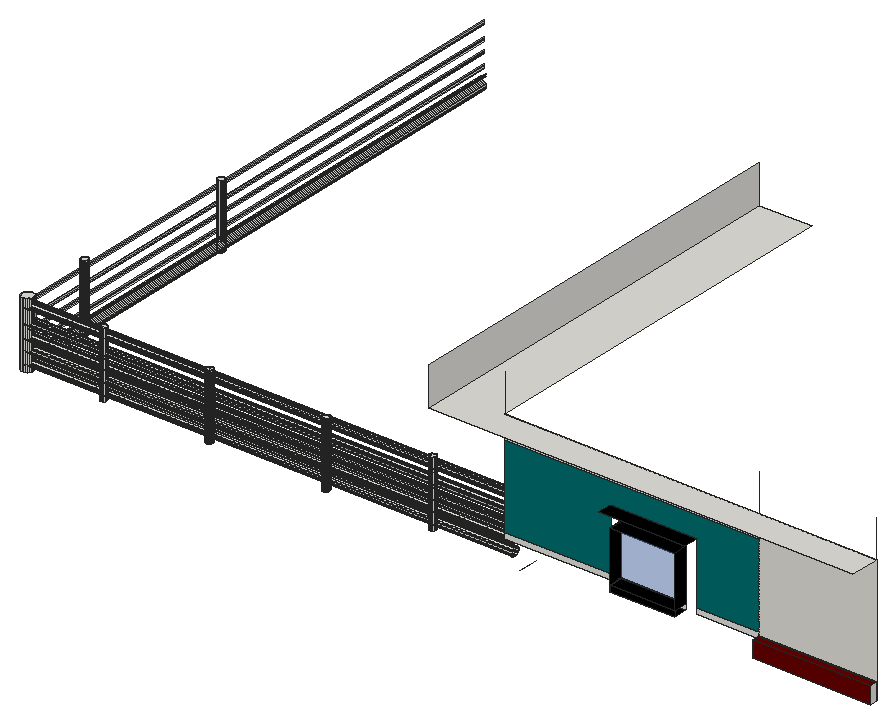
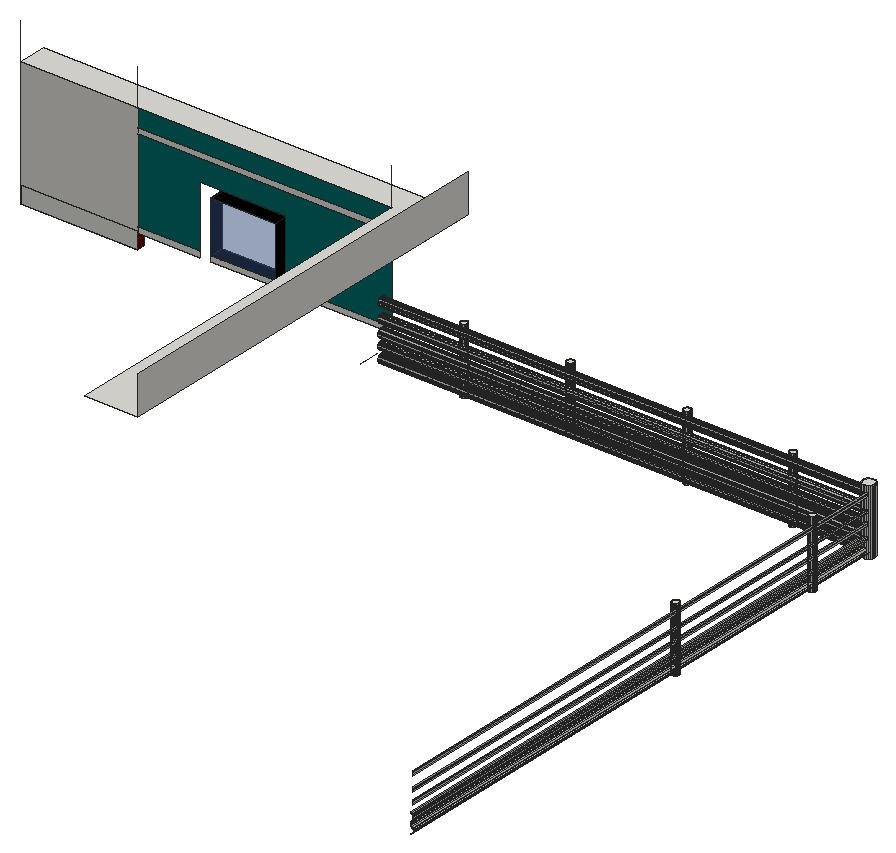
# SketchUp Ruby script. Lengths in inches.
U = 1.inch
M = Sketchup.active_model
def pt(a) = Geom::Point3d.new(a.map { |v| v * U })
def face(e, loops, mat)
  f = e.add_face(loops[0].map { |a| pt(a) })
  loops[1..].each { |l| e.add_face(l.map { |a| pt(a) }).erase! }
  f.material = f.back_material = mat if mat
  f
end
# faces: each face lists its corners as indices into pts; further lists are holes
def faces(e, pts, list, mat = nil) = list.each { |f| face(e, (f[0].is_a?(Array) ? f : [f]).map { |l| l.map { |i| pts[i] } }, mat) }
# xy, xz, yz: faces in a plane at the given z, y or x. An outline is a flat list of corners, or four numbers for a rectangle; further outlines are holes
def ring(l) = l.size == 4 ? [[l[0], l[1]], [l[2], l[1]], [l[2], l[3]], [l[0], l[3]]] : l.each_slice(2).to_a
def flat(e, list, mat, &to3) = list.each { |f| face(e, (f[0].is_a?(Array) ? f : [f]).map { |l| ring(l).map { |u, v| to3.(u, v) } }, mat) }
def xy(e, z, list, mat = nil) = flat(e, list, mat) { |x, y| [x, y, z] }
def xz(e, y, list, mat = nil) = flat(e, list, mat) { |x, z| [x, y, z] }
def yz(e, x, list, mat = nil) = flat(e, list, mat) { |y, z| [x, y, z] }
def lines(e, pts, list) = list.each { |a, b| e.add_line(pt(pts[a]), pt(pts[b])) }
# prism: a flat outline (further loops are holes) pulled along v
def prism(e, loops, v, mat = nil)
  f = face(e, loops, mat); d = Geom::Vector3d.new(v.map { |x| x * U })
  f.pushpull(f.normal.samedirection?(d) ? d.length : -d.length)
end
def box(e, o, s, mat = nil) = prism(e, [[o, [o[0] + s[0], o[1], o[2]], [o[0] + s[0], o[1] + s[1], o[2]], [o[0], o[1] + s[1], o[2]]]], [0, 0, s[2]], mat)
def at(x, y, z, deg = 0) = Geom::Transformation.translation(pt([x, y, z])) * Geom::Transformation.rotation(ORIGIN, Z_AXIS, deg.degrees)
def axes(o, x, y, z) = Geom::Transformation.new([*x, 0, *y, 0, *z, 0, *pt(o).to_a, 1])
def part(name) = M.definitions.add(name)
# library, detail: a bought-in or finely detailed component or shape, given as its bounding box
def library(name, o, s) = part(name).tap { |d| box(d.entities, o, s) }
def detail(e, o, s) = box(e.add_group.entities, o, s)
def put(e, d, t, mat = nil) = e.add_instance(d, t).tap { |i| i.material = mat if mat }
def group(e, t, mat = nil) = e.add_group.tap { |g| g.transformation = t; g.material = mat if mat }.entities
root = M.entities
M.materials.add("[Color A08]").color = [102, 0, 0]
M.materials.add("[Color H07]1").color = [0, 109, 109]
M.materials.add("[Color M09]").color = [0, 0, 0]
M.materials.add("[Marble Carrara Gold Floor Tile]").color = [225, 223, 217]
M.materials.add("[Translucent Glass Blue]1").color = [78, 117, 186]
M.materials["[Translucent Glass Blue]1"].alpha = 0.5
prism(root,[[[92.88,148.57,303.61],[93.25,148.53,303.61],[93.6,148.38,303.61],[93.9,148.15,303.61],[94.13,147.86,303.61],[94.27,147.51,303.61],[94.32,147.14,303.61],[94.27,146.76,303.61],[94.13,146.42,303.61],[93.9,146.12,303.61],[93.6,145.89,303.61],[93.25,145.75,303.61],[92.88,145.7,303.61],[92.51,145.75,303.61],[92.16,145.89,303.61],[91.87,146.12,303.61],[91.64,146.42,303.61],[91.49,146.76,303.61],[91.44,147.14,303.61],[91.49,147.51,303.61],[91.64,147.86,303.61],[91.87,148.15,303.61],[92.16,148.38,303.61],[92.51,148.53,303.61]]],[0,0,28.0625])
prism(root,[[[92.88,219.39,303.61],[93.25,219.34,303.61],[93.6,219.19,303.61],[93.9,218.97,303.61],[94.13,218.67,303.61],[94.27,218.32,303.61],[94.32,217.95,303.61],[94.27,217.58,303.61],[94.13,217.23,303.61],[93.9,216.93,303.61],[93.6,216.7,303.61],[93.25,216.5625,303.61],[92.88,216.51,303.61],[92.51,216.5625,303.61],[92.16,216.7,303.61],[91.87,216.93,303.61],[91.64,217.23,303.61],[91.49,217.58,303.61],[91.44,217.95,303.61],[91.49,218.32,303.61],[91.64,218.67,303.61],[91.87,218.97,303.61],[92.16,219.19,303.61],[92.51,219.34,303.61]]],[0,0,26.6875])
xy(root,307.31,[[400.27,109.91,449.03,112.91]],"[Color A08]")
xy(root,313.34,[[343.08,106.91,369.95,112.91]],"[Color M09]")
xy(root,314.2,[[400.27,109.91,449.03,112.91]],"[Color A08]")
xy(root,315.72,[[343.08,106.91,369.95,112.91]],"[Color M09]")
xy(root,330.8,[[218.35,114.24,218.72,114.29,219.07,114.44,219.36,114.66,219.59,114.96,219.74,115.31,219.78,115.68,219.74,116.05,219.59,116.4,219.36,116.7,219.07,116.93,218.72,117.07,218.35,117.12,217.97,117.07,217.63,116.93,217.33,116.7,217.1,116.4,216.96,116.05,216.91,115.68,216.96,115.31,217.1,114.96,217.33,114.66,217.63,114.44,217.97,114.29],[168.99,115.46,169.36,115.51,169.71,115.65,170,115.88,170.23,116.18,170.375,116.52,170.43,116.89,170.375,117.27,170.23,117.61,170,117.91,169.71,118.14,169.36,118.28,168.99,118.33,168.62,118.28,168.27,118.14,167.97,117.91,167.74,117.61,167.6,117.27,167.55,116.89,167.6,116.52,167.74,116.18,167.97,115.88,168.27,115.65,168.62,115.51],[261.41,115.74,261.78,115.79,262.13,115.94,262.43,116.16,262.65,116.46,262.8,116.81,262.85,117.18,262.8,117.55,262.65,117.9,262.43,118.2,262.13,118.43,261.78,118.57,261.41,118.62,261.04,118.57,260.69,118.43,260.39,118.2,260.16,117.9,260.02,117.55,259.97,117.18,260.02,116.81,260.16,116.46,260.39,116.16,260.69,115.94,261.04,115.79],[124.66,115.87,125.03,115.92,125.38,116.06,125.68,116.29,125.9,116.59,126.05,116.93,126.1,117.31,126.05,117.68,125.9,118.02,125.68,118.32,125.38,118.55,125.03,118.69,124.66,118.74,124.29,118.69,123.94,118.55,123.64,118.32,123.41,118.02,123.27,117.68,123.22,117.31,123.27,116.93,123.41,116.59,123.64,116.29,123.94,116.06,124.29,115.92]])
xy(root,330.99,[[93.07,115.34,93.69,115.5,94.24,115.82,94.7,116.26,95.02,116.8125,95.1875,117.43,95.19,118.0625,95.03,118.68,94.72,119.23,94.27,119.69,93.72,120.01,93.11,120.18,92.47,120.18,91.85,120.02,91.3,119.7,90.85,119.26,90.53,118.71,90.36,118.1,90.35,117.46,90.51,116.84,90.83,116.29,91.28,115.84,91.82,115.52,92.4375,115.35]])
xy(root,337.01,[[343.08,106.91,369.95,112.91]],"[Color M09]")
xy(root,341.53,[[338.5625,106.91,374.46,112.91]],"[Color M09]")
xy(root,359.87,[[272.85,100.91,272.85,272.1,294.79,272.1,294.79,112.91,449.03,112.91,449.03,100.91]],"[Marble Carrara Gold Floor Tile]")
xz(root,106.91,[[343.08,313.34,369.95,315.72]],"[Color M09]")
xz(root,109.91,[[400.27,307.31,449.03,314.2]],"[Color A08]")
xz(root,112.91,[[400.27,307.31,449.03,314.2],[294.79,313.34,338.5625,315.72],[343.08,313.34,369.95,315.72],[374.46,313.34,400.27,315.72],[294.79,350.34,400.27,352.72]])
xz(root,112.91,[[294.79,315.72,338.5625,315.72,338.5625,341.53,374.46,341.53,374.46,315.72,400.27,315.72,400.27,350.34,294.79,350.34],[294.79,352.72,400.27,359.87]],"[Color H07]1")
xz(root,112.91,[[400.27,314.2,449.03,359.87]],"[Marble Carrara Gold Floor Tile]")
xz(root,112.91,[[343.08,315.72,369.95,337.01]],"[Translucent Glass Blue]1")
xz(root,118.05,[[93.38,304.44,93.84,304.5,94.26,304.68,94.62,304.96,94.9,305.32,95.07,305.74,95.13,306.19,95.07,306.65,94.9,307.07,94.62,307.43,94.26,307.71,93.84,307.88,93.38,307.94,92.93,307.88,92.51,307.71,92.15,307.43,91.87,307.07,91.69,306.65,91.63,306.19,91.69,305.74,91.87,305.32,92.15,304.96,92.51,304.68,92.93,304.5]])
xz(root,120.18,[[92.47,303.61,93.11,330.99]])
yz(root,91.69,[[118.2,309.59,117.75,309.65,117.33,309.82,116.96,310.1,116.6875,310.47,116.51,310.89,116.45,311.34,116.51,311.79,116.6875,312.22,116.96,312.58,117.33,312.86,117.75,313.03,118.2,313.09,118.65,313.03,119.08,312.86,119.4375,312.58,119.72,312.22,119.89,311.79,119.91,311.65,119.95,311.34,119.89,310.89,119.83,310.75,119.72,310.47,119.4375,310.1,119.08,309.82,118.65,309.65],[118.2,314.15,117.75,314.21,117.33,314.39,116.96,314.67,116.6875,315.03,116.51,315.45,116.45,315.9,116.51,316.36,116.6875,316.78,116.96,317.14,117.33,317.42,117.75,317.59,118.2,317.65,118.65,317.59,119.08,317.42,119.42,317.15,119.4375,317.14,119.72,316.78,119.89,316.36,119.91,316.25,119.95,315.9,119.89,315.45,119.72,315.03,119.4375,314.67,119.08,314.39,118.65,314.21],[118.2,319.59,117.75,319.65,117.33,319.82,116.96,320.1,116.6875,320.47,116.51,320.89,116.45,321.34,116.51,321.79,116.6875,322.22,116.96,322.58,117.33,322.86,117.75,323.03,118.2,323.09,118.65,323.03,119.08,322.86,119.4375,322.58,119.72,322.22,119.87,321.84,119.89,321.79,119.95,321.34,119.9,320.9375,119.89,320.89,119.72,320.47,119.4375,320.1,119.08,319.82,118.65,319.65],[118.2,325.72,117.75,325.77,117.33,325.95,116.96,326.23,116.6875,326.59,116.51,327.01,116.45,327.47,116.51,327.92,116.6875,328.34,116.96,328.7,117.33,328.98,117.75,329.16,118.2,329.22,118.65,329.16,119.08,328.98,119.4375,328.7,119.72,328.34,119.87,327.97,119.89,327.92,119.95,327.47,119.9,327.0625,119.89,327.01,119.72,326.59,119.4375,326.23,119.08,325.95,118.65,325.77]])
yz(root,92.15,[[118.2,304.65,117.75,304.71,117.33,304.89,116.96,305.17,116.6875,305.53,116.51,305.95,116.45,306.4,116.51,306.86,116.6875,307.28,116.96,307.64,117.33,307.92,117.75,308.09,118.2,308.15,118.65,308.09,119.08,307.92,119.4375,307.64,119.6,307.43,119.72,307.28,119.89,306.86,119.95,306.4,119.89,305.95,119.72,305.53,119.4375,305.17,119.17,304.96,119.08,304.89,118.65,304.71]])
yz(root,272.85,[[100.91,359.87,272.1,375.61]],"[Marble Carrara Gold Floor Tile]")
yz(root,343.08,[[106.91,313.34,112.91,315.72]])
yz(root,343.08,[[106.91,315.72,112.91,337.01]],"[Color M09]")
yz(root,369.95,[[106.91,315.72,112.91,337.01]],"[Color M09]")
yz(root,400.27,[[109.91,307.31,112.91,313.34],[109.91,313.34,112.91,314.2]],"[Color A08]")
yz(root,449.03,[[109.91,307.31,112.91,314.2]])
p = [[217.97,114.29,303.61],[218.35,114.24,303.61],[218.35,114.24,330.8],[217.97,114.29,330.8],[218.72,114.29,303.61],[218.72,114.29,330.8],
  [217.63,114.44,303.61],[217.63,114.44,330.8],[219.07,114.44,303.61],[219.07,114.44,330.8],[217.33,114.66,303.61],[217.33,114.66,330.8],
  [219.36,114.66,303.61],[219.36,114.66,330.8],[217.1,114.96,303.61],[217.1,114.96,330.8],[219.59,114.96,303.61],[219.59,114.96,330.8],
  [216.96,115.31,303.61],[216.96,115.31,330.8],[219.74,115.31,303.61],[219.74,115.31,330.8],[91.82,115.52,303.61],[92.4375,115.35,303.61],
  [92.4375,115.35,330.99],[91.82,115.52,330.99],[93.07,115.34,303.61],[93.07,115.34,330.99],[93.69,115.5,303.61],[93.69,115.5,330.99],
  [216.91,115.68,303.61],[216.91,115.68,330.8],[219.78,115.68,303.61],[219.78,115.68,330.8],[91.28,115.84,303.61],[91.28,115.84,330.99],
  [94.24,115.82,303.61],[94.24,115.82,330.99],[168.27,115.65,303.61],[168.62,115.51,303.61],[168.62,115.51,330.8],[168.27,115.65,330.8],
  [168.99,115.46,303.61],[168.99,115.46,330.8],[169.36,115.51,303.61],[169.36,115.51,330.8],[169.71,115.65,303.61],[169.71,115.65,330.8],
  [167.97,115.88,303.61],[167.97,115.88,330.8],[170,115.88,303.61],[170,115.88,330.8],[216.96,116.05,303.61],[216.96,116.05,330.8],
  [219.74,116.05,303.61],[219.74,116.05,330.8],[261.04,115.79,303.61],[261.41,115.74,303.61],[261.41,115.74,330.8],[261.04,115.79,330.8],
  [261.78,115.79,303.61],[261.78,115.79,330.8],[90.83,116.29,303.61],[90.83,116.29,330.99],[94.7,116.26,303.61],[94.7,116.26,330.99],
  [260.69,115.94,303.61],[260.69,115.94,330.8],[262.13,115.94,303.61],[262.13,115.94,330.8],[123.94,116.06,303.61],[124.29,115.92,303.61],
  [124.29,115.92,330.8],[123.94,116.06,330.8],[124.66,115.87,303.61],[124.66,115.87,330.8],[125.03,115.92,303.61],[125.03,115.92,330.8],
  [125.38,116.06,303.61],[125.38,116.06,330.8],[167.74,116.18,303.61],[167.74,116.18,330.8],[170.23,116.18,303.61],[170.23,116.18,330.8],
  [260.39,116.16,303.61],[260.39,116.16,330.8],[262.43,116.16,303.61],[262.43,116.16,330.8],[123.64,116.29,303.61],[123.64,116.29,330.8],
  [125.68,116.29,303.61],[125.68,116.29,330.8],[217.1,116.4,303.61],[217.1,116.4,330.8],[219.59,116.4,303.61],[219.59,116.4,330.8],
  [167.6,116.52,303.61],[167.6,116.52,330.8],[170.375,116.52,303.61],[170.375,116.52,330.8],[260.16,116.46,303.61],[260.16,116.46,330.8],
  [262.65,116.46,303.61],[262.65,116.46,330.8],[90.51,116.84,303.61],[90.51,116.84,330.99],[95.02,116.8125,303.61],[95.02,116.8125,330.99],
  [123.41,116.59,303.61],[123.41,116.59,330.8],[125.9,116.59,303.61],[125.9,116.59,330.8],[217.33,116.7,303.61],[217.33,116.7,330.8],
  [219.36,116.7,303.61],[219.36,116.7,330.8],[167.55,116.89,303.61],[167.55,116.89,330.8],[170.43,116.89,303.61],[170.43,116.89,330.8],
  [260.02,116.81,303.61],[260.02,116.81,330.8],[262.8,116.81,303.61],[262.8,116.81,330.8],[123.27,116.93,303.61],[123.27,116.93,330.8],
  [126.05,116.93,303.61],[126.05,116.93,330.8],[217.63,116.93,303.61],[217.63,116.93,330.8],[219.07,116.93,303.61],[219.07,116.93,330.8],
  [90.35,117.46,303.61],[90.35,117.46,330.99],[95.1875,117.43,303.61],[95.1875,117.43,330.99],[259.97,117.18,303.61],[259.97,117.18,330.8],
  [262.85,117.18,303.61],[262.85,117.18,330.8],[123.22,117.31,303.61],[123.22,117.31,330.8],[126.1,117.31,303.61],[126.1,117.31,330.8],
  [167.6,117.27,303.61],[167.6,117.27,330.8],[170.375,117.27,303.61],[170.375,117.27,330.8],[217.97,117.07,303.61],[217.97,117.07,330.8],
  [218.72,117.07,303.61],[218.72,117.07,330.8],[218.35,117.12,303.61],[218.35,117.12,330.8],[260.02,117.55,303.61],[260.02,117.55,330.8],
  [262.8,117.55,303.61],[262.8,117.55,330.8],[123.27,117.68,303.61],[123.27,117.68,330.8],[126.05,117.68,303.61],[126.05,117.68,330.8],
  [167.74,117.61,303.61],[167.74,117.61,330.8],[170.23,117.61,303.61],[170.23,117.61,330.8],[95.19,118.0625,303.61],[95.19,118.0625,330.99],
  [90.36,118.1,303.61],[90.36,118.1,330.99],[167.97,117.91,303.61],[167.97,117.91,330.8],[170,117.91,303.61],[170,117.91,330.8],
  [260.16,117.9,303.61],[260.16,117.9,330.8],[262.65,117.9,303.61],[262.65,117.9,330.8],[123.41,118.02,303.61],[123.41,118.02,330.8],
  [125.9,118.02,303.61],[125.9,118.02,330.8],[168.27,118.14,303.61],[168.27,118.14,330.8],[169.71,118.14,303.61],[169.71,118.14,330.8],
  [260.39,118.2,303.61],[260.39,118.2,330.8],[262.43,118.2,303.61],[262.43,118.2,330.8],[123.64,118.32,303.61],[123.64,118.32,330.8],
  [125.68,118.32,303.61],[125.68,118.32,330.8],[90.53,118.71,303.61],[90.53,118.71,330.99],[95.03,118.68,303.61],[95.03,118.68,330.99],
  [168.62,118.28,303.61],[168.62,118.28,330.8],[169.36,118.28,303.61],[169.36,118.28,330.8],[260.69,118.43,303.61],[260.69,118.43,330.8],
  [262.13,118.43,303.61],[262.13,118.43,330.8],[123.94,118.55,303.61],[123.94,118.55,330.8],[125.38,118.55,303.61],[125.38,118.55,330.8],
  [168.99,118.33,303.61],[168.99,118.33,330.8],[261.04,118.57,303.61],[261.04,118.57,330.8],[261.78,118.57,303.61],[261.78,118.57,330.8],
  [124.29,118.69,303.61],[124.29,118.69,330.8],[125.03,118.69,303.61],[125.03,118.69,330.8],[261.41,118.62,303.61],[261.41,118.62,330.8],
  [90.85,119.26,303.61],[90.85,119.26,330.99],[94.72,119.23,303.61],[94.72,119.23,330.99],[124.66,118.74,303.61],[124.66,118.74,330.8],
  [94.27,119.69,303.61],[94.27,119.69,330.99],[91.3,119.7,303.61],[91.3,119.7,330.99],[91.85,120.02,303.61],[91.85,120.02,330.99],
  [93.72,120.01,303.61],[93.72,120.01,330.99],[92.47,120.18,303.61],[92.47,120.18,330.99],[93.11,120.18,303.61],[93.11,120.18,330.99],
  [92.93,118.05,304.5],[92.93,352.8,304.5],[93.38,352.8,304.44],[93.38,118.05,304.44],[93.84,352.8,304.5],[93.84,118.05,304.5],
  [94.26,352.8,304.68],[94.26,118.05,304.68],[294.79,117.75,304.71],[294.79,117.33,304.89],[92.15,117.33,304.89],[92.15,117.75,304.71],
  [294.79,118.2,304.65],[92.15,118.2,304.65],[92.15,355.8,304.96],[92.51,355.8,304.68],[92.51,118.05,304.68],[92.15,118.05,304.96],
  [92.15,119.17,304.96],[94.62,352.8,304.96],[94.62,118.05,304.96],[294.79,118.65,304.71],[92.15,118.65,304.71],[294.79,119.08,304.89],
  [92.15,119.08,304.89],[294.79,116.96,305.17],[92.15,116.96,305.17],[294.79,119.4375,305.17],[92.15,119.4375,305.17],[91.87,355.8,305.32],
  [91.87,118.05,305.32],[94.9,352.8,305.32],[94.9,118.05,305.32],[294.79,116.6875,305.53],[92.15,116.6875,305.53],[294.79,119.72,305.53],
  [92.15,119.72,305.53],[95.07,352.8,305.74],[95.07,118.05,305.74],[294.79,116.51,305.95],[92.15,116.51,305.95],[294.79,119.89,305.95],
  [92.15,119.89,305.95],[95.13,352.8,306.19],[95.13,118.05,306.19],[294.79,116.45,306.4],[92.15,116.45,306.4],[294.79,119.95,306.4],
  [92.15,119.95,306.4],[95.07,352.8,306.65],[95.07,118.05,306.65],[294.79,116.51,306.86],[92.15,116.51,306.86],[294.79,119.89,306.86],
  [92.15,119.89,306.86],[94.9,352.8,307.07],[94.9,118.05,307.07],[294.79,116.6875,307.28],[92.15,116.6875,307.28],[294.79,119.72,307.28],
  [92.15,119.72,307.28],[92.15,355.8,307.43],[91.87,355.8,307.07],[91.87,118.05,307.07],[92.15,118.05,307.43],[92.15,119.6,307.43],
  [94.62,352.8,307.43],[94.62,118.05,307.43],[294.79,116.96,307.64],[92.15,116.96,307.64],[294.79,119.4375,307.64],[92.15,119.4375,307.64],
  [92.51,355.8,307.71],[92.51,118.05,307.71],[94.26,352.8,307.71],[94.26,118.05,307.71],[294.79,117.33,307.92],[92.15,117.33,307.92],
  [294.79,119.08,307.92],[92.15,119.08,307.92],[93.84,352.8,307.88],[93.84,118.05,307.88],[294.79,117.75,308.09],[92.15,117.75,308.09],
  [93.38,118.05,307.94],[93.38,352.8,307.94],[92.93,352.8,307.88],[92.93,118.05,307.88],[294.79,118.65,308.09],[92.15,118.65,308.09],
  [294.79,118.2,308.15],[92.15,118.2,308.15],[92.93,118.05,309.51],[92.93,352.8,309.51],[93.38,352.8,309.45],[93.38,118.05,309.45],
  [93.84,352.8,309.51],[93.84,118.05,309.51],[94.26,352.8,309.6875],[94.26,118.05,309.6875],[294.79,117.75,309.65],[294.79,117.33,309.82],
  [91.69,117.33,309.82],[91.69,117.75,309.65],[294.79,118.2,309.59],[91.69,118.2,309.59],[294.79,118.65,309.65],[91.69,118.65,309.65],
  [294.79,119.08,309.82],[91.69,119.08,309.82],[94.62,352.8,309.96],[94.62,118.05,309.96],[294.79,116.96,310.1],[91.69,116.96,310.1],
  [294.79,119.4375,310.1],[91.69,119.4375,310.1],[94.9,352.8,310.33],[94.9,118.05,310.33],[294.79,116.6875,310.47],[91.69,116.6875,310.47],
  [294.79,119.72,310.47],[91.69,119.72,310.47],[91.69,355.8,310.75],[91.87,355.8,310.33],[91.87,118.05,310.33],[91.69,118.05,310.75],
  [91.69,119.83,310.75],[95.07,352.8,310.75],[95.07,118.05,310.75],[294.79,116.51,310.89],[91.69,116.51,310.89],[294.79,119.89,310.89],
  [91.69,119.89,310.89],[91.63,355.8,311.2],[91.63,118.05,311.2],[294.79,116.45,311.34],[91.69,116.45,311.34],[294.79,119.95,311.34],
  [91.69,119.95,311.34],[91.69,355.8,311.65],[91.69,118.05,311.65],[91.69,119.91,311.65],[294.79,116.51,311.79],[91.69,116.51,311.79],
  [294.79,119.89,311.79],[91.69,119.89,311.79],[91.87,355.8,312.08],[91.87,118.05,312.08],[294.79,116.6875,312.22],[91.69,116.6875,312.22],
  [294.79,119.72,312.22],[91.69,119.72,312.22],[294.79,116.96,312.58],[91.69,116.96,312.58],[294.79,119.4375,312.58],[91.69,119.4375,312.58],
  [294.79,117.33,312.86],[91.69,117.33,312.86],[294.79,119.08,312.86],[91.69,119.08,312.86],[294.79,117.75,313.03],[91.69,117.75,313.03],
  [294.79,118.65,313.03],[91.69,118.65,313.03],[294.79,118.2,313.09],[91.69,118.2,313.09],[294.79,117.75,314.21],[294.79,117.33,314.39],
  [91.69,117.33,314.39],[91.69,117.75,314.21],[294.79,118.2,314.15],[91.69,118.2,314.15],[294.79,118.65,314.21],[91.69,118.65,314.21],
  [294.79,119.08,314.39],[91.69,119.08,314.39],[294.79,116.96,314.67],[91.69,116.96,314.67],[294.79,119.4375,314.67],[91.69,119.4375,314.67],
  [294.79,116.6875,315.03],[91.69,116.6875,315.03],[294.79,119.72,315.03],[91.69,119.72,315.03],[294.79,116.51,315.45],[91.69,116.51,315.45],
  [294.79,119.89,315.45],[91.69,119.89,315.45],[294.79,116.45,315.9],[91.69,116.45,315.9],[294.79,119.95,315.9],[91.69,119.95,315.9],
  [91.69,355.8,316.25],[91.87,355.8,315.83],[91.87,118.05,315.83],[91.69,118.05,316.25],[91.69,119.91,316.25],[294.79,116.51,316.36],
  [91.69,116.51,316.36],[294.79,119.89,316.36],[91.69,119.89,316.36],[91.63,355.8,316.7],[91.63,118.05,316.7],[294.79,116.6875,316.78],
  [91.69,116.6875,316.78],[294.79,119.72,316.78],[91.69,119.72,316.78],[91.69,355.8,317.15],[91.69,118.05,317.15],[91.69,119.42,317.15],
  [294.79,116.96,317.14],[91.69,116.96,317.14],[294.79,119.4375,317.14],[91.69,119.4375,317.14],[294.79,117.33,317.42],[91.69,117.33,317.42],
  [294.79,119.08,317.42],[91.69,119.08,317.42],[91.87,355.8,317.58],[91.87,118.05,317.58],[294.79,117.75,317.59],[91.69,117.75,317.59],
  [294.79,118.65,317.59],[91.69,118.65,317.59],[294.79,118.2,317.65],[91.69,118.2,317.65],[294.79,117.75,319.65],[294.79,117.33,319.82],
  [91.69,117.33,319.82],[91.69,117.75,319.65],[294.79,118.2,319.59],[91.69,118.2,319.59],[294.79,118.65,319.65],[91.69,118.65,319.65],
  [294.79,119.08,319.82],[91.69,119.08,319.82],[294.79,116.96,320.1],[91.69,116.96,320.1],[294.79,119.4375,320.1],[91.69,119.4375,320.1],
  [294.79,116.6875,320.47],[91.69,116.6875,320.47],[294.79,119.72,320.47],[91.69,119.72,320.47],[294.79,116.51,320.89],[91.69,116.51,320.89],
  [91.69,355.8,320.9375],[91.87,355.8,320.51],[91.87,118.05,320.51],[91.69,118.05,320.9375],[91.69,119.9,320.9375],[294.79,119.89,320.89],
  [91.69,119.89,320.89],[294.79,116.45,321.34],[91.69,116.45,321.34],[91.63,355.8,321.39],[91.63,118.05,321.39],[294.79,119.95,321.34],
  [91.69,119.95,321.34],[294.79,116.51,321.79],[91.69,116.51,321.79],[294.79,119.89,321.79],[91.69,119.89,321.79],[91.69,355.8,321.84],
  [91.69,118.05,321.84],[91.69,119.87,321.84],[294.79,116.6875,322.22],[91.69,116.6875,322.22],[91.87,355.8,322.26],[91.87,118.05,322.26],
  [294.79,119.72,322.22],[91.69,119.72,322.22],[294.79,116.96,322.58],[91.69,116.96,322.58],[294.79,119.4375,322.58],[91.69,119.4375,322.58],
  [294.79,117.33,322.86],[91.69,117.33,322.86],[294.79,119.08,322.86],[91.69,119.08,322.86],[294.79,117.75,323.03],[91.69,117.75,323.03],
  [294.79,118.65,323.03],[91.69,118.65,323.03],[294.79,118.2,323.09],[91.69,118.2,323.09],[294.79,118.2,325.72],[294.79,117.75,325.77],
  [91.69,117.75,325.77],[91.69,118.2,325.72],[294.79,118.65,325.77],[91.69,118.65,325.77],[294.79,117.33,325.95],[91.69,117.33,325.95],
  [294.79,119.08,325.95],[91.69,119.08,325.95],[294.79,116.96,326.23],[91.69,116.96,326.23],[294.79,119.4375,326.23],[91.69,119.4375,326.23],
  [294.79,116.6875,326.59],[91.69,116.6875,326.59],[294.79,119.72,326.59],[91.69,119.72,326.59],[294.79,116.51,327.01],[91.69,116.51,327.01],
  [91.69,355.8,327.0625],[91.87,355.8,326.64],[91.87,118.05,326.64],[91.69,118.05,327.0625],[91.69,119.9,327.0625],[294.79,119.89,327.01],
  [91.69,119.89,327.01],[294.79,116.45,327.47],[91.69,116.45,327.47],[294.79,119.95,327.47],[91.69,119.95,327.47],[91.63,355.8,327.51],
  [91.63,118.05,327.51],[294.79,116.51,327.92],[91.69,116.51,327.92],[91.69,355.8,327.97],[91.69,118.05,327.97],[91.69,119.87,327.97],
  [294.79,119.89,327.92],[91.69,119.89,327.92],[294.79,116.6875,328.34],[91.69,116.6875,328.34],[294.79,119.72,328.34],[91.69,119.72,328.34],
  [91.87,355.8,328.39],[91.87,118.05,328.39],[294.79,116.96,328.7],[91.69,116.96,328.7],[294.79,119.4375,328.7],[91.69,119.4375,328.7],
  [294.79,117.33,328.98],[91.69,117.33,328.98],[294.79,119.08,328.98],[91.69,119.08,328.98],[294.79,117.75,329.16],[91.69,117.75,329.16],
  [294.79,118.65,329.16],[91.69,118.65,329.16],[294.79,118.2,329.22],[91.69,118.2,329.22],[300.79,121.91,303.61],[300.79,112.91,303.61],
  [449.03,112.91,359.87],[449.03,112.91,375.61],[294.79,112.91,359.87],[294.79,112.91,375.61],[400.27,112.91,359.87],[400.27,112.91,375.61]]
faces(root,p,[[0,1,2,3],[1,4,5,2],[6,0,3,7],[4,8,9,5],[10,6,7,11],[8,12,13,9],[14,10,11,15],[12,16,17,13],
  [18,14,15,19],[16,20,21,17],[22,23,24,25],[23,26,27,24],[26,28,29,27],[30,18,19,31],[20,32,33,21],[34,22,25,35],
  [28,36,37,29],[38,39,40,41],[39,42,43,40],[42,44,45,43],[44,46,47,45],[48,38,41,49],[46,50,51,47],[52,30,31,53],
  [32,54,55,33],[56,57,58,59],[57,60,61,58],[62,34,35,63],[36,64,65,37],[66,56,59,67],[60,68,69,61],[70,71,72,73],
  [71,74,75,72],[74,76,77,75],[76,78,79,77],[80,48,49,81],[50,82,83,51],[84,66,67,85],[68,86,87,69],[88,70,73,89],
  [78,90,91,79],[92,52,53,93],[54,94,95,55],[96,80,81,97],[82,98,99,83],[100,84,85,101],[86,102,103,87],[104,62,63,105],
  [64,106,107,65],[108,88,89,109],[90,110,111,91],[112,92,93,113],[94,114,115,95],[116,96,97,117],[98,118,119,99],[120,100,101,121],
  [102,122,123,103],[124,108,109,125],[110,126,127,111],[128,112,113,129],[114,130,131,115],[132,104,105,133],[106,134,135,107],[136,120,121,137],
  [122,138,139,123],[140,124,125,141],[126,142,143,127],[144,116,117,145],[118,146,147,119],[148,128,129,149],[130,150,151,131],[152,148,149,153],
  [150,152,153,151],[154,136,137,155],[138,156,157,139],[158,140,141,159],[142,160,161,143],[162,144,145,163],[146,164,165,147],[134,166,167,135],
  [168,132,133,169],[170,162,163,171],[164,172,173,165],[174,154,155,175],[156,176,177,157],[178,158,159,179],[160,180,181,161],[182,170,171,183],
  [172,184,185,173],[186,174,175,187],[176,188,189,177],[190,178,179,191],[180,192,193,181],[194,168,169,195],[166,196,197,167],[198,182,183,199],
  [184,200,201,185],[202,186,187,203],[188,204,205,189],[206,190,191,207],[192,208,209,193],[210,198,199,211],[200,210,211,201],[212,202,203,213],
  [204,214,215,205],[216,206,207,217],[208,218,219,209],[220,212,213,221],[214,220,221,215],[222,194,195,223],[196,224,225,197],[226,216,217,227],
  [218,226,227,219],[224,228,229,225],[230,222,223,231],[232,230,231,233],[228,234,235,229],[236,232,233,237],[234,238,239,235],[240,241,242,243],
  [243,242,244,245],[245,244,246,247],[248,249,250,251],[252,248,251,253],[254,255,256,257,258],[247,246,259,260],[261,252,253,262],[263,261,262,264],
  [249,265,266,250],[267,263,264,258,268],[269,254,258,257,270],[260,259,271,272],[265,273,274,266],[275,267,268,276],[272,271,277,278],[273,279,280,274],
  [281,275,276,282],[278,277,283,284],[279,285,286,280],[287,281,282,288],[284,283,289,290],[285,291,292,286],[293,287,288,294],[290,289,295,296],
  [291,297,298,292],[299,293,294,300],[301,302,303,304,305],[296,295,306,307],[297,308,309,298],[310,299,300,305,311],[312,301,305,304,313],[307,306,314,315],
  [308,316,317,309],[318,310,311,319],[315,314,320,321],[316,322,323,317],[324,325,326,327],[321,320,325,324],[328,318,319,329],[322,330,331,323],
  [330,328,329,331],[332,333,334,335],[335,334,336,337],[337,336,338,339],[340,341,342,343],[344,340,343,345],[346,344,345,347],[348,346,347,349],
  [339,338,350,351],[341,352,353,342],[354,348,349,355],[351,350,356,357],[352,358,359,353],[360,354,355,361],[362,363,364,365,366],[357,356,367,368],
  [358,369,370,359],[371,360,361,366,372],[373,362,366,365,374],[369,375,376,370],[377,371,372,378],[379,373,374,380,381],[375,382,383,376],[384,377,378,381,385],
  [386,379,381,380,387],[382,388,389,383],[390,384,385,391],[388,392,393,389],[394,390,391,395],[392,396,397,393],[398,394,395,399],[396,400,401,397],
  [402,398,399,403],[400,404,405,401],[404,402,403,405],[406,407,408,409],[410,406,409,411],[412,410,411,413],[414,412,413,415],[407,416,417,408],
  [418,414,415,419],[416,420,421,417],[422,418,419,423],[420,424,425,421],[426,422,423,427],[424,428,429,425],[430,426,427,431],[432,433,434,435,436],
  [428,437,438,429],[439,430,431,436,440],[441,432,436,435,442],[437,443,444,438],[445,439,440,446],[447,441,442,448,449],[443,450,451,444],[452,445,446,453],
  [450,454,455,451],[456,452,453,449,457],[458,447,449,448,459],[454,460,461,455],[462,456,457,463],[460,464,465,461],[464,462,463,465],[466,467,468,469],
  [470,466,469,471],[472,470,471,473],[474,472,473,475],[467,476,477,468],[478,474,475,479],[476,480,481,477],[482,478,479,483],[480,484,485,481],
  [486,487,488,489,490],[491,482,483,492],[484,493,494,485],[495,486,490,489,496],[497,491,492,490,498],[493,499,500,494],[501,497,498,502],[503,495,496,504,505],
  [499,506,507,500],[508,503,505,504,509],[510,501,502,505,511],[506,512,513,507],[514,510,511,515],[512,516,517,513],[518,514,515,519],[516,520,521,517],
  [522,518,519,523],[520,524,525,521],[524,522,523,525],[526,527,528,529],[530,526,529,531],[527,532,533,528],[534,530,531,535],[532,536,537,533],
  [538,534,535,539],[536,540,541,537],[542,538,539,543],[540,544,545,541],[546,547,548,549,550],[551,542,543,552],[544,553,554,545],[555,551,552,550,556],
  [557,546,550,549,558],[553,559,560,554],[561,557,558,562,563],[564,555,556,565],[559,566,567,560],[568,564,565,563,569],[570,561,563,562,571],[566,572,573,567],
  [574,568,569,575],[572,576,577,573],[578,574,575,579],[576,580,581,577],[582,578,579,583],[580,584,585,581],[584,582,583,585]])
lines(root,p,[[586,587],[588,589],[590,591],[592,593]])
